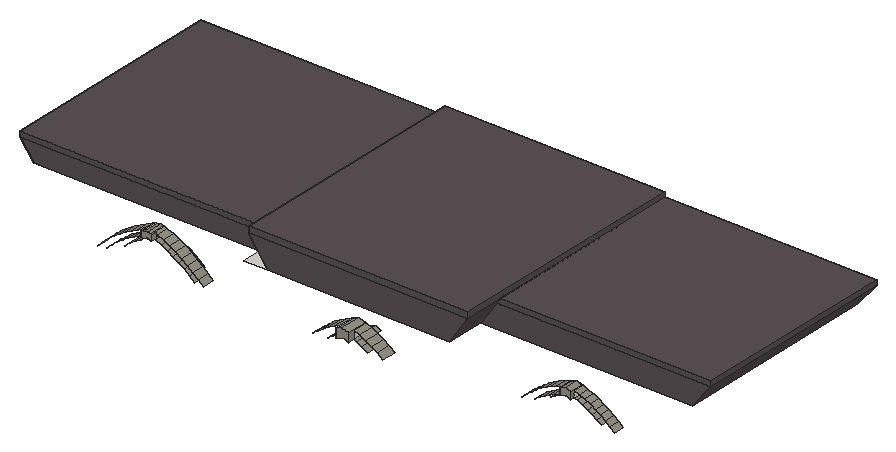
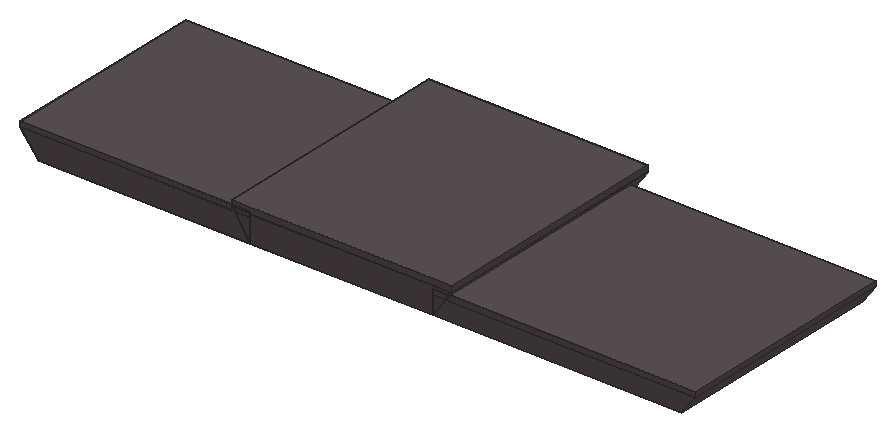
# SketchUp Ruby script. Lengths in inches.
U = 1.inch
M = Sketchup.active_model
def pt(a) = Geom::Point3d.new(a.map { |v| v * U })
def face(e, loops, mat)
  f = e.add_face(loops[0].map { |a| pt(a) })
  loops[1..].each { |l| e.add_face(l.map { |a| pt(a) }).erase! }
  f.material = f.back_material = mat if mat
  f
end
# faces: each face lists its corners as indices into pts; further lists are holes
def faces(e, pts, list, mat = nil) = list.each { |f| face(e, (f[0].is_a?(Array) ? f : [f]).map { |l| l.map { |i| pts[i] } }, mat) }
# xy, xz, yz: faces in a plane at the given z, y or x. An outline is a flat list of corners, or four numbers for a rectangle; further outlines are holes
def ring(l) = l.size == 4 ? [[l[0], l[1]], [l[2], l[1]], [l[2], l[3]], [l[0], l[3]]] : l.each_slice(2).to_a
def flat(e, list, mat, &to3) = list.each { |f| face(e, (f[0].is_a?(Array) ? f : [f]).map { |l| ring(l).map { |u, v| to3.(u, v) } }, mat) }
def xy(e, z, list, mat = nil) = flat(e, list, mat) { |x, y| [x, y, z] }
def xz(e, y, list, mat = nil) = flat(e, list, mat) { |x, z| [x, y, z] }
def yz(e, x, list, mat = nil) = flat(e, list, mat) { |y, z| [x, y, z] }
def lines(e, pts, list) = list.each { |a, b| e.add_line(pt(pts[a]), pt(pts[b])) }
# prism: a flat outline (further loops are holes) pulled along v
def prism(e, loops, v, mat = nil)
  f = face(e, loops, mat); d = Geom::Vector3d.new(v.map { |x| x * U })
  f.pushpull(f.normal.samedirection?(d) ? d.length : -d.length)
end
def box(e, o, s, mat = nil) = prism(e, [[o, [o[0] + s[0], o[1], o[2]], [o[0] + s[0], o[1] + s[1], o[2]], [o[0], o[1] + s[1], o[2]]]], [0, 0, s[2]], mat)
def at(x, y, z, deg = 0) = Geom::Transformation.translation(pt([x, y, z])) * Geom::Transformation.rotation(ORIGIN, Z_AXIS, deg.degrees)
def axes(o, x, y, z) = Geom::Transformation.new([*x, 0, *y, 0, *z, 0, *pt(o).to_a, 1])
def part(name) = M.definitions.add(name)
# library, detail: a bought-in or finely detailed component or shape, given as its bounding box
def library(name, o, s) = part(name).tap { |d| box(d.entities, o, s) }
def detail(e, o, s) = box(e.add_group.entities, o, s)
def put(e, d, t, mat = nil) = e.add_instance(d, t).tap { |i| i.material = mat if mat }
def group(e, t, mat = nil) = e.add_group.tap { |g| g.transformation = t; g.material = mat if mat }.entities
root = M.entities
M.materials.add("[Asphalt New]").color = [91, 82, 84]
M.materials.add("[Formica Graystone]").color = [149, 146, 135]
M.materials.add("[Terrazzo Tile Light]1").color = [219, 217, 210]
xy(root,647.54,[[101.22,131.66,102.84,135.04]],"[Formica Graystone]")
xy(root,647.8,[[108.86,131.66,110.11,135.04]],"[Formica Graystone]")
xy(root,652.04,[[101.22,131.66,102.84,135.04]],"[Formica Graystone]")
xy(root,652.33,[[108.86,131.66,110.11,135.04]],"[Formica Graystone]")
xy(root,660.875,[[199.67,128.91,317.75,144.04],[317.75,128.91,338.35,144.04],[10.25,144.04,30.78,144.04,30.78,301.14,199.67,301.14,199.67,315.41,10.25,315.41],[30.78,144.04,181.54,301.14],[181.54,144.04,199.67,148.61],
  [199.67,144.04,317.75,301.14],[317.75,144.04,338.35,301.14],[181.54,148.61,199.67,158.3],[181.54,158.3,199.67,301.14],[338.35,158.3,483.98,301.14],
  [483.98,158.3,499.12,158.3,499.12,315.41,338.35,315.41,338.35,301.14,483.98,301.14],[199.67,301.14,338.35,315.41]])
xy(root,660.875,[[181.54,128.91,199.67,144.04]],"[Terrazzo Tile Light]1")
xy(root,674.625,[[0,144.04,199.67,315.41]])
xy(root,678.5625,[[338.35,158.3,512.93,315.41]])
xy(root,679,[[0,144.04,199.67,315.41]],"[Asphalt New]")
xy(root,681.1875,[[185.55,128.91,352.17,315.41]])
xy(root,682.625,[[338.35,158.3,512.93,315.41]],"[Asphalt New]")
xy(root,685.875,[[185.55,128.91,352.17,315.41]],"[Asphalt New]")
xz(root,128.04,[[252.55,633.7,254.87,634.75,257.4,635.71,259.96,634.83,262.125,633.92,262.125,640.46,257.3,642.13,252.55,640.31]],"[Formica Graystone]")
xz(root,128.91,[[199.67,660.875,338.35,660.875,352.17,681.1875,185.55,681.1875,185.55,680.625],[185.55,681.1875,352.17,685.875]],"[Asphalt New]")
xz(root,131.66,[[101.22,647.54,102.84,647.54,106.32,648.74,108.86,647.8,110.11,647.8,110.11,652.33,108.86,652.33,106.37,653.25,102.84,652.04,101.22,652.04]],"[Formica Graystone]")
xz(root,135.04,[[101.22,647.54,102.84,647.54,102.84,652.04,101.35,651.53,101.22,651.47],[108.86,647.8,110.11,647.8,110.11,651.87,108.86,652.33],[101.22,651.47,101.22,652.04,102.84,652.04,101.35,651.53],[110.11,651.87,108.86,652.33,110.11,652.33]])
xz(root,144.04,[[252.55,633.7,252.55,640.31,257.3,642.13,262.125,640.46,262.125,633.92,259.96,634.83,257.4,635.71,254.87,634.75],[102.84,647.54,102.84,652.04,106.37,653.25,108.86,652.33,108.86,647.8,106.32,648.74]])
xz(root,144.04,[[10.25,660.875,199.67,660.875,199.67,674.625,0,674.625],[0,674.625,199.67,679]],"[Asphalt New]")
xz(root,147.55,[[406.79,640.32,408.37,640.9,411.11,641.74,413.85,640.92,415.41,640.35,415.41,645.63,411.09,646.9375,406.79,645.61]],"[Formica Graystone]")
xz(root,158.3,[[406.79,640.32,406.79,645.61,411.09,646.9375,415.41,645.63,415.41,640.35,413.85,640.92,411.11,641.74,408.37,640.9]])
xz(root,158.3,[[338.35,660.875,499.12,660.875,512.93,678.5625,338.35,678.5625],[338.35,678.5625,512.93,682.625]],"[Asphalt New]")
xz(root,315.41,[[10.25,660.875,0,674.625,189.84,674.625,199.67,660.875],[199.67,660.875,199.67,679,186.71,679,185.55,680.625,338.35,680.625,338.35,660.875],[199.67,660.875,189.84,674.625,199.67,674.625],[338.35,660.875,338.35,678.5625,350.38,678.5625],[338.35,660.875,350.38,678.5625,512.93,678.5625,499.12,660.875],
  [0,674.625,0,679,186.71,679,189.84,674.625],[189.84,674.625,186.71,679,189.84,679],[189.84,674.625,199.67,679],[338.35,678.5625,350.38,681.1875],[350.38,678.5625,350.38,681.1875,352.17,681.1875],
  [350.38,678.5625,352.17,681.1875,352.17,682.625,512.93,682.625,512.93,678.5625],[185.55,680.625,338.35,681.1875],[185.55,681.1875,185.55,685.875,352.17,685.875,352.17,682.625,338.35,682.625,338.35,681.1875],[338.35,681.1875,350.38,682.625],[350.38,681.1875,352.17,682.625]],"[Asphalt New]")
yz(root,0,[[144.04,674.625,315.41,679]],"[Asphalt New]")
yz(root,101.22,[[131.66,647.54,135.04,652.04]],"[Formica Graystone]")
yz(root,102.84,[[135.04,647.54,144.04,652.04]])
yz(root,108.86,[[135.04,647.8,144.04,652.33]])
yz(root,110.11,[[131.66,647.8,135.04,652.33]],"[Formica Graystone]")
yz(root,185.55,[[128.91,680.625,315.41,681.1875],[128.91,681.1875,315.41,685.875]],"[Asphalt New]")
yz(root,199.67,[[144.04,660.875,315.41,674.625],[144.04,674.625,315.41,679]])
yz(root,252.55,[[128.04,633.7,132.97,640.31],[132.97,633.7,144.04,640.31]])
yz(root,262.125,[[132.97,633.92,144.04,640.46]])
yz(root,262.125,[[128.04,633.92,132.97,640.46]],"[Formica Graystone]")
yz(root,338.35,[[158.3,660.875,315.41,678.5625],[158.3,678.5625,315.41,682.625]])
yz(root,352.17,[[128.91,681.1875,315.41,685.875]],"[Asphalt New]")
yz(root,406.79,[[150.49,640.32,158.3,645.61]])
yz(root,406.79,[[147.55,640.32,150.49,645.61]],"[Formica Graystone]")
yz(root,415.41,[[150.49,640.35,158.3,645.63]])
yz(root,415.41,[[147.55,640.35,150.49,645.63]],"[Formica Graystone]")
yz(root,512.93,[[158.3,678.5625,315.41,682.625]],"[Asphalt New]")
p = [[234.87,144.04,630.33],[230.86,144.04,627.2],[230.86,132.97,627.2],[234.87,132.97,630.33],[379.39,158.3,630.31],[376.01,158.3,627.33],
  [376.01,150.49,627.33],[379.39,150.49,630.31],[446.21,158.3,627.37],[442.83,158.3,630.36],[442.83,150.49,630.36],[446.21,150.49,627.37],
  [284.07,144.04,627.61],[280.04,144.04,630.74],[280.04,132.97,630.74],[284.07,132.97,627.61],[146.23,144.04,627.91],[142.46,144.04,631.63],
  [142.46,135.04,631.63],[146.23,135.04,627.91],[242.33,144.04,628.15],[246.38,144.04,630.6],[246.38,132.97,630.6],[242.33,132.97,628.15],
  [70.05,144.04,631.91],[66.31,144.04,628.13],[66.31,135.04,628.13],[70.05,135.04,631.91],[256.79,144.04,630.13],[252.76,144.04,628.31],
  [252.76,158.91,628.31],[254.77,158.91,629.22],[256.79,158.91,630.13],[132.8,144.04,628.37],[129.02,144.04,631.38],[129.02,153.35,631.38],
  [132.8,153.35,628.37],[268.52,144.04,630.88],[272.59,144.04,628.5],[272.59,132.97,628.5],[268.52,132.97,630.88],[135.76,144.04,631.89],
  [139.55,144.04,628.53],[139.55,135.04,628.53],[135.76,135.04,631.89],[262.22,144.04,628.45],[258.17,144.04,630.16],[258.17,158.91,630.16],
  [259.04,158.91,629.79],[262.22,158.91,628.45],[83.48,144.04,631.7],[79.73,144.04,628.7],[79.73,153.35,628.7],[83.48,153.35,631.7],
  [72.98,144.04,628.83],[76.75,144.04,632.21],[76.75,135.04,632.21],[72.98,135.04,628.83],[394.63,158.3,631.03],[391.18,158.3,628.86],
  [391.18,166.11,628.86],[394.63,166.11,631.03],[431.04,158.3,628.92],[427.6,158.3,631.09],[427.6,166.11,631.09],[431.04,166.11,628.92],
  [385.91,158.3,629.12],[389.375,158.3,631.57],[389.375,150.49,631.57],[385.91,150.49,629.12],[432.85,158.3,631.625],[436.32,158.3,629.17],
  [436.32,150.49,629.17],[432.85,150.49,631.625],[257.48,144.04,630.4],[257.48,158.91,630.4],[239.06,144.04,633.22],[239.06,132.97,633.22],
  [382.93,158.3,633.1],[382.93,150.49,633.1],[439.29,158.3,633.15],[439.29,150.49,633.15],[250.5625,144.04,632.8],[250.5625,132.97,632.8],
  [275.81,144.04,633.61],[275.81,132.97,633.61],[264.31,144.04,632.99],[264.31,132.97,632.99],[398.18,158.3,633.02],[398.18,166.11,633.02],
  [424.05,158.3,633.07],[424.05,166.11,633.07],[125.09,144.04,634.18],[125.09,153.35,634.18],[138.5,144.04,635.15],[138.5,135.04,635.15],
  [392.97,158.3,633.83],[392.97,150.49,633.83],[429.26,158.3,633.89],[429.26,150.49,633.89],[87.39,144.04,634.49],[87.39,153.35,634.49],
  [74,144.04,635.46],[74,135.04,635.46],[131.79,144.04,635.05],[131.79,135.04,635.05],[80.71,144.04,635.38],[80.71,135.04,635.38],
  [252.55,144.04,633.7],[252.55,132.97,633.7],[262.125,144.04,633.92],[262.125,132.97,633.92],[401.84,158.3,634.82],[401.84,166.11,634.82],
  [386.61,158.3,635.7],[386.61,150.49,635.7],[420.39,158.3,634.85],[420.39,166.11,634.85],[243.41,144.04,635.85],[243.41,132.97,635.85],
  [435.61,158.3,635.76],[435.61,150.49,635.76],[271.4,144.04,636.1875],[271.4,132.97,636.1875],[254.87,144.04,634.75],[254.87,128.04,634.75],
  [252.55,128.04,633.7],[396.67,158.3,635.9],[396.67,150.49,635.9],[259.96,144.04,634.83],[262.125,128.04,633.92],[259.96,128.04,634.83],
  [425.55,158.3,635.95],[425.55,150.49,635.95],[121.02,144.04,636.77],[121.02,153.35,636.77],[91.46,144.04,637.04],[91.46,153.35,637.04],
  [257.4,144.04,635.71],[257.4,128.04,635.71],[405.59,158.3,636.42],[405.59,166.11,636.42],[416.65,158.3,636.44],[416.65,166.11,636.44],
  [127.66,144.04,638],[127.66,135.04,638],[134.35,144.04,638.45],[134.35,135.04,638.45],[84.84,144.04,638.3125],[84.84,135.04,638.3125],
  [78.15,144.04,638.78],[78.15,135.04,638.78],[390.43,158.3,638.1],[390.43,150.49,638.1],[247.91,144.04,638.22],[247.91,132.97,638.22],
  [431.8,158.3,638.16],[431.8,150.49,638.16],[400.48,158.3,637.77],[400.48,150.49,637.77],[421.74,158.3,637.81],[421.74,150.49,637.81],
  [266.83,144.04,638.48],[266.83,132.97,638.48],[409.41,158.3,637.82],[407.5,166.11,637.12],[409.41,166.11,637.82],[412.82,158.3,637.83],
  [412.82,166.11,637.83],[116.8125,144.04,639.14],[116.8125,153.35,639.14],[95.67,144.04,639.35],[95.67,153.35,639.35],[404.39,158.3,639.44],
  [404.39,150.49,639.44],[417.84,158.3,639.47],[417.84,150.49,639.47],[411.11,158.3,638.34],[411.11,166.11,638.34],[411.64,166.11,638.18],
  [123.38,144.04,640.72],[123.38,135.04,640.72],[394.36,158.3,640.3],[394.36,150.49,640.3],[252.55,144.04,640.31],[252.55,132.97,640.31],
  [427.86,158.3,640.36],[427.86,150.49,640.36],[89.13,144.04,641],[89.13,135.04,641],[130.04,144.04,641.52],[130.04,135.04,641.52],
  [262.125,144.04,640.46],[262.125,132.97,640.46],[82.48,144.04,641.85],[82.48,135.04,641.85],[112.49,144.04,641.28],[112.49,153.35,641.28],
  [100.01,144.04,641.42],[100.01,153.35,641.42],[406.79,158.3,640.32],[406.79,150.49,640.32],[415.41,158.3,640.35],[415.41,150.49,640.35],
  [257.3,144.04,642.13],[252.55,128.04,640.31],[257.3,128.04,642.13],[408.37,158.3,640.9],[408.37,147.55,640.9],[406.79,147.55,640.32],
  [413.85,158.3,640.92],[415.41,147.55,640.35],[413.85,147.55,640.92],[398.41,158.3,642.29],[398.41,150.49,642.29],[423.8,158.3,642.34],
  [423.8,150.49,642.34],[262.125,128.04,640.46],[118.97,144.04,643.21],[118.97,135.04,643.21],[411.11,158.3,641.74],[411.11,147.55,641.74],
  [93.58,144.04,643.45],[93.58,135.04,643.45],[108.06,144.04,643.19],[108.06,153.35,643.19],[104.46,144.04,643.23],[103.16,153.35,642.71],
  [104.46,153.35,643.23],[125.57,144.04,644.37],[125.57,135.04,644.37],[86.98,144.04,644.67],[86.98,135.04,644.67],[402.55,158.3,644.0625],
  [402.55,150.49,644.0625],[419.65,158.3,644.1],[419.65,150.49,644.1],[114.42,144.04,645.46],[114.42,135.04,645.46],[106.26,144.04,643.85],
  [106.26,153.35,643.85],[107.82,153.35,643.28],[98.15,144.04,645.63],[98.15,135.04,645.63],[406.79,158.3,645.61],[406.79,150.49,645.61],
  [415.41,158.3,645.63],[415.41,150.49,645.63],[120.95,144.04,646.97],[120.95,135.04,646.97],[91.63,144.04,647.23],[91.63,135.04,647.23],
  [109.76,144.04,647.46],[109.76,135.04,647.46],[102.84,144.04,647.54],[102.84,135.04,647.54],[411.09,158.3,646.9375],[406.79,147.55,645.61],
  [411.09,147.55,646.9375],[415.41,147.55,645.63],[116.21,144.04,649.32],[116.21,135.04,649.32],[96.43,144.04,649.52],[96.43,135.04,649.52],
  [106.32,144.04,648.74],[106.32,131.66,648.74],[102.84,131.66,647.54],[108.86,144.04,647.8],[108.86,135.04,647.8],[108.86,131.66,647.8],
  [111.34,144.04,651.41],[111.34,135.04,651.41],[101.35,144.04,651.53],[101.22,135.04,651.47],[101.35,135.04,651.53],[108.86,144.04,652.33],
  [108.86,135.04,652.33],[110.11,135.04,651.87],[102.84,144.04,652.04],[102.84,135.04,652.04],[106.37,144.04,653.25],[102.84,131.66,652.04],
  [106.37,131.66,653.25],[108.86,131.66,652.33],[199.67,128.91,660.875],[185.55,128.91,680.625],[185.55,315.41,680.625],[186.71,315.41,679],
  [189.84,315.41,674.625],[199.67,315.41,660.875],[199.67,301.14,660.875],[199.67,158.3,660.875],[199.67,148.61,660.875],[199.67,144.04,660.875],
  [352.17,128.91,681.1875],[338.35,128.91,660.875],[338.35,144.04,660.875],[338.35,158.3,660.875],[338.35,301.14,660.875],[338.35,315.41,660.875],
  [350.38,315.41,678.5625],[352.17,315.41,681.1875],[10.25,144.04,660.875],[0,144.04,674.625],[0,315.41,674.625],[10.25,315.41,660.875],
  [512.93,158.3,678.5625],[499.12,158.3,660.875],[499.12,315.41,660.875],[512.93,315.41,678.5625],[415.41,158.3,640.32]]
faces(root,p,[[0,1,2,3],[4,5,6,7],[8,9,10,11],[12,13,14,15],[16,17,18,19],[20,21,22,23],[24,25,26,27],[28,29,30,31,32],
  [33,34,35,36],[37,38,39,40],[41,42,43,44],[45,46,47,48,49],[50,51,52,53],[54,55,56,57],[58,59,60,61],[62,63,64,65],
  [66,67,68,69],[70,71,72,73],[74,28,32,75],[46,74,75,47],[76,0,3,77],[78,4,7,79],[9,80,81,10],[21,82,83,22],
  [13,84,85,14],[86,37,40,87],[88,58,61,89],[63,90,91,64],[34,92,93,35],[17,94,95,18],[67,96,97,68],[98,70,73,99],
  [100,50,53,101],[102,24,27,103],[104,41,44,105],[55,106,107,56],[82,108,109,83],[110,86,87,111],[112,88,89,113],[114,78,79,115],
  [90,116,117,91],[118,76,77,119],[80,120,121,81],[84,122,123,85],[108,124,125,126,109],[96,127,128,97],[129,110,111,130,131],[132,98,99,133],
  [92,134,135,93],[136,100,101,137],[124,138,139,125],[138,129,131,139],[140,112,113,141],[116,142,143,117],[144,104,105,145],[94,146,147,95],
  [106,148,149,107],[150,102,103,151],[152,114,115,153],[154,118,119,155],[120,156,157,121],[127,158,159,128],[160,132,133,161],[122,162,163,123],
  [164,140,141,165,166],[142,167,168,143],[134,169,170,135],[171,136,137,172],[158,173,174,159],[175,160,161,176],[177,164,166,178],[167,177,178,179,168],
  [180,144,145,181],[182,152,153,183],[184,154,155,185],[156,186,187,157],[148,188,189,149],[146,190,191,147],[162,192,193,163],[194,150,151,195],
  [169,196,197,170],[198,171,172,199],[173,200,201,174],[202,175,176,203],[204,184,185,205,206],[200,207,208,209,201],[210,202,203,211,212],[213,182,183,214],
  [186,215,216,187],[192,204,206,217,193],[218,180,181,219],[207,220,221,208],[220,210,212,221],[188,222,223,189],[196,224,225,197],[226,198,199,227,228],
  [190,229,230,191],[231,194,195,232],[233,213,214,234],[215,235,236,216],[237,218,219,238],[239,226,228,240],[224,239,240,241,225],[222,242,243,223],
  [244,233,234,245],[235,246,247,236],[229,248,249,230],[250,231,232,251],[252,237,238,253],[242,254,255,243],[256,244,245,257,258],[246,256,258,259,247],
  [248,260,261,249],[262,250,251,263],[254,264,265,266,255],[267,252,253,268],[264,267,268,269,265],[260,270,271,261],[272,262,263,273,274],[270,275,276,277,271],
  [278,272,274,279],[280,278,279,281,282],[275,280,282,283,276]],"[Formica Graystone]")
faces(root,p,[[284,285,286,287,288,289,290,291,292,293],[294,295,296,297,298,299,300,301],[302,303,304,305],[306,307,308,309]],"[Asphalt New]")
lines(root,p,[[202,310]])
